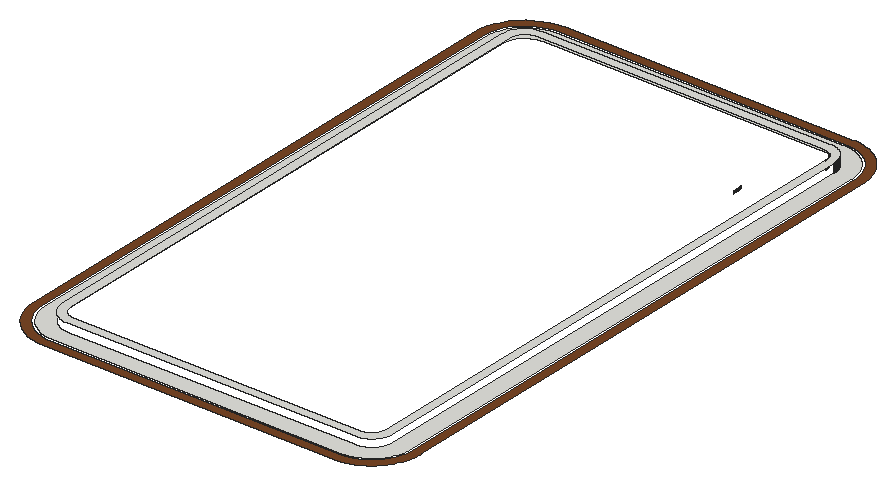
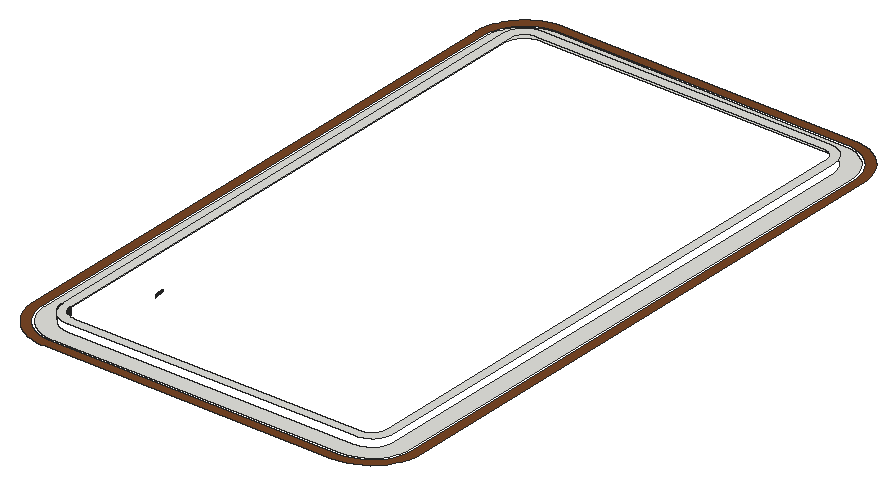
# SketchUp Ruby script. Lengths in inches.
U = 1.inch
M = Sketchup.active_model
def pt(a) = Geom::Point3d.new(a.map { |v| v * U })
def face(e, loops, mat)
  f = e.add_face(loops[0].map { |a| pt(a) })
  loops[1..].each { |l| e.add_face(l.map { |a| pt(a) }).erase! }
  f.material = f.back_material = mat if mat
  f
end
# faces: each face lists its corners as indices into pts; further lists are holes
def faces(e, pts, list, mat = nil) = list.each { |f| face(e, (f[0].is_a?(Array) ? f : [f]).map { |l| l.map { |i| pts[i] } }, mat) }
# xy, xz, yz: faces in a plane at the given z, y or x. An outline is a flat list of corners, or four numbers for a rectangle; further outlines are holes
def ring(l) = l.size == 4 ? [[l[0], l[1]], [l[2], l[1]], [l[2], l[3]], [l[0], l[3]]] : l.each_slice(2).to_a
def flat(e, list, mat, &to3) = list.each { |f| face(e, (f[0].is_a?(Array) ? f : [f]).map { |l| ring(l).map { |u, v| to3.(u, v) } }, mat) }
def xy(e, z, list, mat = nil) = flat(e, list, mat) { |x, y| [x, y, z] }
def xz(e, y, list, mat = nil) = flat(e, list, mat) { |x, z| [x, y, z] }
def yz(e, x, list, mat = nil) = flat(e, list, mat) { |y, z| [x, y, z] }
def lines(e, pts, list) = list.each { |a, b| e.add_line(pt(pts[a]), pt(pts[b])) }
# prism: a flat outline (further loops are holes) pulled along v
def prism(e, loops, v, mat = nil)
  f = face(e, loops, mat); d = Geom::Vector3d.new(v.map { |x| x * U })
  f.pushpull(f.normal.samedirection?(d) ? d.length : -d.length)
end
def box(e, o, s, mat = nil) = prism(e, [[o, [o[0] + s[0], o[1], o[2]], [o[0] + s[0], o[1] + s[1], o[2]], [o[0], o[1] + s[1], o[2]]]], [0, 0, s[2]], mat)
def at(x, y, z, deg = 0) = Geom::Transformation.translation(pt([x, y, z])) * Geom::Transformation.rotation(ORIGIN, Z_AXIS, deg.degrees)
def axes(o, x, y, z) = Geom::Transformation.new([*x, 0, *y, 0, *z, 0, *pt(o).to_a, 1])
def part(name) = M.definitions.add(name)
# library, detail: a bought-in or finely detailed component or shape, given as its bounding box
def library(name, o, s) = part(name).tap { |d| box(d.entities, o, s) }
def detail(e, o, s) = box(e.add_group.entities, o, s)
def put(e, d, t, mat = nil) = e.add_instance(d, t).tap { |i| i.material = mat if mat }
def group(e, t, mat = nil) = e.add_group.tap { |g| g.transformation = t; g.material = mat if mat }.entities
root = M.entities
M.materials.add("[Wood Veneer 01]3").color = [120, 70, 37]
xy(root,121,[[[75.09,29.75,144.24,29.75,144.36,29.76,144.48,29.76,144.6,29.77,144.73,29.78,144.97,29.8,145.09,29.8125,145.21,29.83,145.33,29.85,145.45,29.86,145.57,29.88,145.6875,29.9,145.8,29.93,145.92,29.95,146.16,30.01,146.28,30.03,146.39,30.07,146.63,30.13,146.74,30.17,146.86,30.2,146.97,30.24,147.09,30.28,147.31,30.36,147.43,30.41,147.54,30.45,148.09,30.7,148.2,30.76,148.31,30.8125,148.41,30.87,148.52,30.93,148.73,31.05,148.83,31.11,148.9375,31.18,149.04,31.24,149.14,31.31,149.24,31.375,149.34,31.45,149.4375,31.52,149.53,31.59,149.63,31.66,149.73,31.74,149.82,31.8125,149.91,31.89,150.01,31.97,150.1,32.05,150.1875,32.125,150.28,32.21,150.37,32.29,150.45,32.375,150.54,32.46,150.625,32.55,150.71,32.63,150.79,32.72,150.875,32.8125,150.95,32.9,151.03,32.99,151.11,33.09,151.1875,33.18,151.26,33.27,151.34,33.37,151.41,33.47,151.48,33.5625,151.55,33.66,151.625,33.76,151.69,33.86,151.76,33.96,151.82,34.0625,151.89,34.17,151.95,34.27,152.07,34.48,152.13,34.59,152.1875,34.69,152.24,34.8,152.3,34.91,152.55,35.46,152.59,35.57,152.64,35.69,152.72,35.91,152.76,36.03,152.8,36.14,152.83,36.26,152.87,36.37,152.93,36.61,152.97,36.72,152.99,36.84,153.05,37.08,153.07,37.2,153.1,37.3125,153.12,37.43,153.14,37.55,153.15,37.67,153.17,37.79,153.1875,37.91,153.2,38.03,153.22,38.27,153.23,38.4,153.24,38.52,153.24,38.64,153.25,38.76,153.25,171.24,153.24,171.36,153.24,171.48,153.23,171.6,153.22,171.73,153.2,171.97,153.1875,172.09,153.17,172.21,153.15,172.33,153.14,172.45,153.12,172.57,153.1,172.6875,153.07,172.8,153.05,172.92,152.99,173.16,152.97,173.28,152.93,173.39,152.87,173.63,152.83,173.74,152.8,173.86,152.76,173.97,152.72,174.09,152.64,174.31,152.59,174.43,152.55,174.54,152.3,175.09,152.24,175.2,152.1875,175.31,152.13,175.41,152.07,175.52,151.95,175.73,151.89,175.83,151.82,175.9375,151.76,176.04,151.69,176.14,151.625,176.24,151.55,176.34,151.48,176.4375,151.41,176.53,151.34,176.63,151.26,176.73,151.1875,176.82,151.11,176.91,151.03,177.01,150.95,177.1,150.875,177.1875,150.79,177.28,150.71,177.37,150.625,177.45,150.54,177.54,150.45,177.625,150.37,177.71,150.28,177.79,150.1875,177.875,150.1,177.95,150.01,178.03,149.91,178.11,149.82,178.1875,149.73,178.26,149.63,178.34,149.53,178.41,149.4375,178.48,149.34,178.55,149.24,178.625,149.14,178.69,149.04,178.76,148.9375,178.82,148.83,178.89,148.73,178.95,148.52,179.07,148.41,179.13,148.31,179.1875,148.2,179.24,148.09,179.3,147.54,179.55,147.43,179.59,147.31,179.64,147.09,179.72,146.97,179.76,146.86,179.8,146.74,179.83,146.63,179.87,146.39,179.93,146.28,179.97,146.16,179.99,145.92,180.05,145.8,180.07,145.6875,180.1,145.57,180.12,145.45,180.14,145.33,180.15,145.21,180.17,145.09,180.1875,144.97,180.2,144.73,180.22,144.6,180.23,144.48,180.24,144.36,180.24,144.24,180.25,75.09,180.25,73.79,180.17,72.61,179.93,71.46,179.54,70.38,179.01,69.37,178.33,68.46,177.54,67.67,176.63,66.99,175.62,66.46,174.54,66.07,173.39,65.83,172.21,65.75,170.91,65.75,39.09,65.83,37.79,66.07,36.61,66.46,35.46,66.99,34.38,67.67,33.37,68.46,32.46,69.37,31.67,70.38,30.99,71.46,30.46,72.61,30.07,73.79,29.83],[75.22,33.75,74.32,33.81,73.64,33.94,73,34.16,72.38,34.47,71.8125,34.85,71.3,35.3,70.85,35.8125,70.47,36.38,70.16,37,69.94,37.64,69.81,38.32,69.75,39.22,69.75,170.78,69.81,171.68,69.94,172.36,70.16,173,70.47,173.62,70.85,174.1875,71.3,174.7,71.8125,175.15,72.38,175.53,73,175.84,73.64,176.06,74.32,176.19,75.22,176.25,144.21,176.25,144.27,176.24,144.34,176.24,144.41,176.23,144.48,176.23,144.69,176.2,144.75,176.2,144.82,176.19,144.89,176.17,144.96,176.16,145.02,176.15,145.09,176.14,145.23,176.1,145.29,176.09,145.43,176.05,145.49,176.03,145.56,176.01,145.62,175.99,145.6875,175.97,145.75,175.95,145.82,175.93,145.88,175.9,145.95,175.875,146.01,175.85,146.07,175.82,146.14,175.8,146.44,175.65,146.51,175.61,146.57,175.58,146.625,175.55,146.68,175.51,146.74,175.48,146.86,175.4,146.92,175.37,146.97,175.33,147.09,175.25,147.14,175.21,147.2,175.16,147.3,175.08,147.36,175.04,147.41,174.99,147.46,174.95,147.51,174.9,147.5625,174.86,147.61,174.81,147.81,174.61,147.86,174.5625,147.9,174.51,147.95,174.46,147.99,174.41,148.04,174.36,148.08,174.3,148.16,174.2,148.21,174.14,148.25,174.09,148.33,173.97,148.37,173.92,148.4,173.86,148.48,173.74,148.51,173.68,148.55,173.625,148.58,173.57,148.61,173.51,148.65,173.44,148.8,173.14,148.82,173.07,148.85,173.01,148.875,172.95,148.9,172.88,148.93,172.82,148.95,172.75,148.97,172.6875,148.99,172.62,149.01,172.56,149.03,172.49,149.05,172.43,149.09,172.29,149.1,172.23,149.14,172.09,149.15,172.02,149.16,171.96,149.17,171.89,149.19,171.82,149.2,171.75,149.2,171.69,149.23,171.48,149.23,171.41,149.24,171.34,149.24,171.27,149.25,171.21,149.25,38.79,149.24,38.73,149.24,38.66,149.23,38.59,149.23,38.52,149.2,38.31,149.2,38.25,149.19,38.18,149.17,38.11,149.16,38.04,149.15,37.98,149.14,37.91,149.1,37.77,149.09,37.71,149.05,37.57,149.03,37.51,149.01,37.44,148.99,37.38,148.97,37.3125,148.95,37.25,148.93,37.18,148.9,37.12,148.875,37.05,148.85,36.99,148.82,36.93,148.8,36.86,148.65,36.56,148.61,36.49,148.58,36.43,148.55,36.375,148.51,36.32,148.48,36.26,148.4,36.14,148.37,36.08,148.33,36.03,148.25,35.91,148.21,35.86,148.16,35.8,148.08,35.7,148.04,35.64,147.99,35.59,147.95,35.54,147.9,35.49,147.86,35.4375,147.81,35.39,147.61,35.19,147.5625,35.14,147.51,35.1,147.46,35.05,147.41,35.01,147.36,34.96,147.3,34.92,147.2,34.84,147.14,34.79,147.09,34.75,146.97,34.67,146.92,34.63,146.86,34.6,146.74,34.52,146.68,34.49,146.625,34.45,146.57,34.42,146.51,34.39,146.44,34.35,146.14,34.2,146.07,34.18,146.01,34.15,145.95,34.125,145.88,34.1,145.82,34.07,145.75,34.05,145.6875,34.03,145.62,34.01,145.56,33.99,145.49,33.97,145.43,33.95,145.29,33.91,145.23,33.9,145.09,33.86,145.02,33.85,144.96,33.84,144.89,33.83,144.82,33.81,144.75,33.8,144.69,33.8,144.48,33.77,144.41,33.77,144.34,33.76,144.27,33.76,144.21,33.75]]])
xy(root,121,[[[75,27,144.3125,27,144.47,27.01,144.63,27.02,144.78,27.03,145.1,27.05,145.25,27.07,145.41,27.08,145.57,27.1,145.72,27.125,145.88,27.15,146.03,27.17,146.1875,27.2,146.34,27.23,146.49,27.26,146.65,27.3,146.8,27.33,146.95,27.37,147.11,27.41,147.41,27.49,147.86,27.64,148.01,27.6875,148.15,27.74,148.3,27.8,148.45,27.85,148.59,27.91,148.74,27.97,148.88,28.04,149.02,28.1,149.17,28.17,149.73,28.45,149.86,28.53,150,28.61,150.14,28.6875,150.27,28.77,150.4,28.85,150.54,28.9375,150.67,29.02,150.93,29.2,151.05,29.29,151.18,29.38,151.31,29.48,151.43,29.58,151.55,29.67,151.67,29.77,151.91,29.98,152.03,30.08,152.15,30.1875,152.26,30.3,152.375,30.4,152.49,30.51,152.6,30.625,152.7,30.74,152.8125,30.85,152.92,30.97,153.02,31.09,153.23,31.33,153.33,31.45,153.42,31.57,153.52,31.69,153.62,31.82,153.71,31.95,153.8,32.07,153.98,32.33,154.0625,32.46,154.15,32.6,154.23,32.73,154.3125,32.86,154.39,33,154.47,33.14,154.55,33.27,154.83,33.83,154.9,33.98,154.96,34.12,155.03,34.26,155.09,34.41,155.15,34.55,155.2,34.7,155.26,34.85,155.3125,34.99,155.36,35.14,155.51,35.59,155.59,35.89,155.63,36.05,155.67,36.2,155.7,36.35,155.74,36.51,155.77,36.66,155.8,36.8125,155.83,36.97,155.85,37.12,155.875,37.28,155.9,37.43,155.92,37.59,155.93,37.75,155.95,37.9,155.97,38.22,155.98,38.37,155.99,38.53,156,38.6875,156,171.3125,155.99,171.47,155.98,171.63,155.97,171.78,155.95,172.1,155.93,172.25,155.92,172.41,155.9,172.57,155.875,172.72,155.85,172.88,155.83,173.03,155.8,173.1875,155.77,173.34,155.74,173.49,155.7,173.65,155.67,173.8,155.63,173.95,155.59,174.11,155.51,174.41,155.36,174.86,155.3125,175.01,155.26,175.15,155.2,175.3,155.15,175.45,155.09,175.59,155.03,175.74,154.96,175.88,154.9,176.02,154.83,176.17,154.55,176.73,154.47,176.86,154.39,177,154.3125,177.14,154.23,177.27,154.15,177.4,154.0625,177.54,153.98,177.67,153.8,177.93,153.71,178.05,153.62,178.18,153.52,178.31,153.42,178.43,153.33,178.55,153.23,178.67,153.02,178.91,152.92,179.03,152.8125,179.15,152.7,179.26,152.6,179.375,152.49,179.49,152.375,179.6,152.26,179.7,152.15,179.8125,152.03,179.92,151.91,180.02,151.67,180.23,151.55,180.33,151.43,180.42,151.31,180.52,151.18,180.62,151.05,180.71,150.93,180.8,150.67,180.98,150.54,181.0625,150.4,181.15,150.27,181.23,150.14,181.3125,150,181.39,149.86,181.47,149.73,181.55,149.17,181.83,149.02,181.9,148.88,181.96,148.74,182.03,148.59,182.09,148.45,182.15,148.3,182.2,148.15,182.26,148.01,182.3125,147.86,182.36,147.41,182.51,147.11,182.59,146.95,182.63,146.8,182.67,146.65,182.7,146.49,182.74,146.34,182.77,146.1875,182.8,146.03,182.83,145.88,182.85,145.72,182.875,145.57,182.9,145.41,182.92,145.25,182.93,145.1,182.95,144.78,182.97,144.63,182.98,144.47,182.99,144.3125,183,75,183,73.43,182.9,71.89,182.59,70.41,182.09,69,181.39,67.69,180.52,66.51,179.49,65.48,178.31,64.61,177,63.91,175.59,63.41,174.11,63.1,172.57,63,171,63,39,63.1,37.43,63.41,35.89,63.91,34.41,64.61,33,65.48,31.69,66.51,30.51,67.69,29.48,69,28.61,70.41,27.91,71.89,27.41,73.43,27.1],[75.07,29,73.7,29.09,72.41,29.34,71.17,29.77,70,30.34,68.91,31.07,67.93,31.93,67.07,32.91,66.34,34,65.77,35.17,65.34,36.41,65.09,37.7,65,39.07,65,170.93,65.09,172.3,65.34,173.59,65.77,174.83,66.34,176,67.07,177.09,67.93,178.07,68.91,178.93,70,179.66,71.17,180.23,72.41,180.66,73.7,180.91,75.07,181,144.26,181,144.39,180.99,144.52,180.99,144.78,180.97,144.92,180.96,145.05,180.95,145.31,180.91,145.43,180.9,145.5625,180.875,145.69,180.86,145.82,180.83,145.95,180.81,146.21,180.75,146.33,180.72,146.59,180.66,146.71,180.625,146.84,180.59,146.97,180.55,147.21,180.47,147.34,180.43,147.46,180.38,147.58,180.34,147.71,180.29,147.83,180.24,147.95,180.1875,148.07,180.14,148.1875,180.08,148.31,180.03,148.42,179.97,148.66,179.85,148.77,179.79,148.89,179.72,149,179.66,149.11,179.59,149.22,179.53,149.34,179.46,149.45,179.39,149.56,179.31,149.66,179.24,149.77,179.17,149.88,179.09,149.98,179.01,150.09,178.93,150.29,178.77,150.39,178.6875,150.49,178.6,150.59,178.52,150.79,178.34,150.88,178.25,150.98,178.16,151.16,177.98,151.25,177.88,151.34,177.79,151.52,177.59,151.6,177.49,151.6875,177.39,151.77,177.29,151.93,177.09,152.01,176.98,152.09,176.88,152.17,176.77,152.24,176.66,152.31,176.56,152.39,176.45,152.46,176.34,152.53,176.22,152.59,176.11,152.66,176,152.72,175.89,152.79,175.77,152.85,175.66,152.97,175.42,153.03,175.31,153.08,175.1875,153.14,175.07,153.1875,174.95,153.24,174.83,153.29,174.71,153.34,174.58,153.38,174.46,153.43,174.34,153.47,174.21,153.55,173.97,153.59,173.84,153.625,173.71,153.66,173.59,153.72,173.33,153.75,173.21,153.81,172.95,153.83,172.82,153.86,172.69,153.875,172.5625,153.9,172.43,153.91,172.31,153.95,172.05,153.96,171.92,153.97,171.78,153.99,171.52,153.99,171.39,154,171.26,154,38.74,153.99,38.61,153.99,38.48,153.97,38.22,153.96,38.08,153.95,37.95,153.91,37.69,153.9,37.57,153.875,37.4375,153.86,37.31,153.83,37.18,153.81,37.05,153.75,36.79,153.72,36.67,153.66,36.41,153.625,36.29,153.59,36.16,153.55,36.03,153.47,35.79,153.43,35.66,153.38,35.54,153.34,35.42,153.29,35.29,153.24,35.17,153.1875,35.05,153.14,34.93,153.08,34.8125,153.03,34.69,152.97,34.58,152.85,34.34,152.79,34.23,152.72,34.11,152.66,34,152.59,33.89,152.53,33.78,152.46,33.66,152.39,33.55,152.31,33.44,152.24,33.34,152.17,33.23,152.09,33.12,152.01,33.02,151.93,32.91,151.77,32.71,151.6875,32.61,151.6,32.51,151.52,32.41,151.34,32.21,151.25,32.12,151.16,32.02,150.98,31.84,150.88,31.75,150.79,31.66,150.59,31.48,150.49,31.4,150.39,31.3125,150.29,31.23,150.09,31.07,149.98,30.99,149.88,30.91,149.77,30.83,149.66,30.76,149.56,30.69,149.45,30.61,149.34,30.54,149.22,30.47,149.11,30.41,149,30.34,148.89,30.28,148.77,30.21,148.66,30.15,148.42,30.03,148.31,29.97,148.1875,29.92,148.07,29.86,147.95,29.8125,147.83,29.76,147.71,29.71,147.58,29.66,147.46,29.62,147.34,29.57,147.21,29.53,146.97,29.45,146.84,29.41,146.71,29.375,146.59,29.34,146.33,29.28,146.21,29.25,145.95,29.19,145.82,29.17,145.69,29.14,145.5625,29.125,145.43,29.1,145.31,29.09,145.05,29.05,144.92,29.04,144.78,29.03,144.52,29.01,144.39,29.01,144.26,29]]],"[Wood Veneer 01]3")
xy(root,123,[[[75.22,33.75,144.21,33.75,144.27,33.76,144.34,33.76,144.41,33.77,144.48,33.77,144.69,33.8,144.75,33.8,144.82,33.81,144.89,33.83,144.96,33.84,145.02,33.85,145.09,33.86,145.23,33.9,145.29,33.91,145.43,33.95,145.49,33.97,145.56,33.99,145.62,34.01,145.6875,34.03,145.75,34.05,145.82,34.07,145.88,34.1,145.95,34.125,146.01,34.15,146.07,34.18,146.14,34.2,146.44,34.35,146.51,34.39,146.57,34.42,146.625,34.45,146.68,34.49,146.74,34.52,146.86,34.6,146.92,34.63,146.97,34.67,147.09,34.75,147.14,34.79,147.2,34.84,147.3,34.92,147.36,34.96,147.41,35.01,147.46,35.05,147.51,35.1,147.5625,35.14,147.61,35.19,147.81,35.39,147.86,35.4375,147.9,35.49,147.95,35.54,147.99,35.59,148.04,35.64,148.08,35.7,148.16,35.8,148.21,35.86,148.25,35.91,148.33,36.03,148.37,36.08,148.4,36.14,148.48,36.26,148.51,36.32,148.55,36.375,148.58,36.43,148.61,36.49,148.65,36.56,148.8,36.86,148.82,36.93,148.85,36.99,148.875,37.05,148.9,37.12,148.93,37.18,148.95,37.25,148.97,37.3125,148.99,37.38,149.01,37.44,149.03,37.51,149.05,37.57,149.09,37.71,149.1,37.77,149.14,37.91,149.15,37.98,149.16,38.04,149.17,38.11,149.19,38.18,149.2,38.25,149.2,38.31,149.23,38.52,149.23,38.59,149.24,38.66,149.24,38.73,149.25,38.79,149.25,171.21,149.24,171.27,149.24,171.34,149.23,171.41,149.23,171.48,149.2,171.69,149.2,171.75,149.19,171.82,149.17,171.89,149.16,171.96,149.15,172.02,149.14,172.09,149.1,172.23,149.09,172.29,149.05,172.43,149.03,172.49,149.01,172.56,148.99,172.62,148.97,172.6875,148.95,172.75,148.93,172.82,148.9,172.88,148.875,172.95,148.85,173.01,148.82,173.07,148.8,173.14,148.65,173.44,148.61,173.51,148.58,173.57,148.55,173.625,148.51,173.68,148.48,173.74,148.4,173.86,148.37,173.92,148.33,173.97,148.25,174.09,148.21,174.14,148.16,174.2,148.08,174.3,148.04,174.36,147.99,174.41,147.95,174.46,147.9,174.51,147.86,174.5625,147.81,174.61,147.61,174.81,147.5625,174.86,147.51,174.9,147.46,174.95,147.41,174.99,147.36,175.04,147.3,175.08,147.2,175.16,147.14,175.21,147.09,175.25,146.97,175.33,146.92,175.37,146.86,175.4,146.74,175.48,146.68,175.51,146.625,175.55,146.57,175.58,146.51,175.61,146.44,175.65,146.14,175.8,146.07,175.82,146.01,175.85,145.95,175.875,145.88,175.9,145.82,175.93,145.75,175.95,145.6875,175.97,145.62,175.99,145.56,176.01,145.49,176.03,145.43,176.05,145.29,176.09,145.23,176.1,145.09,176.14,145.02,176.15,144.96,176.16,144.89,176.17,144.82,176.19,144.75,176.2,144.69,176.2,144.48,176.23,144.41,176.23,144.34,176.24,144.27,176.24,144.21,176.25,75.22,176.25,74.32,176.19,73.64,176.06,73,175.84,72.38,175.53,71.8125,175.15,71.3,174.7,70.85,174.1875,70.47,173.62,70.16,173,69.94,172.36,69.81,171.68,69.75,170.78,69.75,39.22,69.81,38.32,69.94,37.64,70.16,37,70.47,36.38,70.85,35.8125,71.3,35.3,71.8125,34.85,72.38,34.47,73,34.16,73.64,33.94,74.32,33.81],[75.29,35.75,74.58,35.8,74.16,35.88,73.76,36.01,73.38,36.2,73.03,36.4375,72.72,36.72,72.4375,37.03,72.2,37.38,72.01,37.76,71.88,38.16,71.8,38.58,71.75,39.29,71.75,170.71,71.8,171.42,71.88,171.84,72.01,172.24,72.2,172.62,72.4375,172.97,72.72,173.28,73.03,173.5625,73.38,173.8,73.76,173.99,74.16,174.12,74.58,174.2,75.29,174.25,144.17,174.25,144.21,174.24,144.3,174.24,144.34,174.23,144.38,174.23,144.42,174.22,144.47,174.22,144.55,174.2,144.59,174.2,144.63,174.1875,144.68,174.18,144.92,174.12,144.96,174.1,145.04,174.08,145.08,174.0625,145.125,174.05,145.16,174.03,145.2,174.02,145.24,174,145.28,173.99,145.4,173.93,145.4375,173.91,145.48,173.9,145.51,173.875,145.55,173.86,145.59,173.84,145.625,173.8125,145.66,173.79,145.7,173.77,145.73,173.75,145.77,173.73,145.81,173.7,145.84,173.68,145.875,173.65,145.91,173.63,145.94,173.6,145.98,173.58,146.01,173.55,146.05,173.53,146.14,173.44,146.17,173.42,146.21,173.39,146.39,173.21,146.42,173.17,146.44,173.14,146.53,173.05,146.55,173.01,146.58,172.98,146.6,172.94,146.63,172.91,146.65,172.875,146.68,172.84,146.7,172.81,146.73,172.77,146.75,172.73,146.77,172.7,146.79,172.66,146.8125,172.625,146.84,172.59,146.86,172.55,146.875,172.51,146.9,172.48,146.91,172.4375,146.93,172.4,146.99,172.28,147,172.24,147.02,172.2,147.03,172.16,147.05,172.125,147.0625,172.08,147.08,172.04,147.1,171.96,147.12,171.92,147.18,171.68,147.1875,171.63,147.2,171.59,147.2,171.55,147.22,171.47,147.22,171.42,147.23,171.38,147.23,171.34,147.24,171.3,147.24,171.21,147.25,171.17,147.25,38.83,147.24,38.79,147.24,38.7,147.23,38.66,147.23,38.62,147.22,38.58,147.22,38.53,147.2,38.45,147.2,38.41,147.1875,38.37,147.18,38.32,147.12,38.08,147.1,38.04,147.08,37.96,147.0625,37.92,147.05,37.875,147.03,37.84,147.02,37.8,147,37.76,146.99,37.72,146.93,37.6,146.91,37.5625,146.9,37.52,146.875,37.49,146.86,37.45,146.84,37.41,146.8125,37.375,146.79,37.34,146.77,37.3,146.75,37.27,146.73,37.23,146.7,37.19,146.68,37.16,146.65,37.125,146.63,37.09,146.6,37.06,146.58,37.02,146.55,36.99,146.53,36.95,146.44,36.86,146.42,36.83,146.39,36.79,146.21,36.61,146.17,36.58,146.14,36.56,146.05,36.47,146.01,36.45,145.98,36.42,145.94,36.4,145.91,36.37,145.875,36.35,145.84,36.32,145.81,36.3,145.77,36.27,145.73,36.25,145.7,36.23,145.66,36.21,145.625,36.1875,145.59,36.16,145.55,36.14,145.51,36.125,145.48,36.1,145.4375,36.09,145.4,36.07,145.28,36.01,145.24,36,145.2,35.98,145.16,35.97,145.125,35.95,145.08,35.9375,145.04,35.92,144.96,35.9,144.92,35.88,144.68,35.82,144.63,35.8125,144.59,35.8,144.55,35.8,144.47,35.78,144.42,35.78,144.38,35.77,144.34,35.77,144.3,35.76,144.21,35.76,144.17,35.75]]])
yz(root,139.5,[[153,121,153.18,121.5],[153.18,121,153.35,121.5]],"[Wood Veneer 01]3")
yz(root,147.2,[[171.55,121,171.59,123]])
yz(root,147.22,[[171.42,121,171.47,123]])
yz(root,147.23,[[171.34,121,171.38,123]])
yz(root,147.24,[[171.21,121,171.25,123],[171.25,121,171.3,123]])
yz(root,147.25,[[170.97,121,171.04,123],[171.04,121,171.09,123],[171.09,121,171.13,123],[171.13,121,171.17,123]])
yz(root,149.2,[[171.69,121,171.75,123]])
yz(root,149.23,[[171.41,121,171.48,123]])
yz(root,149.24,[[171.27,121,171.34,123]])
yz(root,149.25,[[170.98,121,171.07,123],[171.07,121,171.14,123],[171.14,121,171.21,123]])
p = [[139.5,153.35,121],[139.49,153.53,121],[139.49,153.53,121.5],[139.5,153.35,121.5],[139.48,153.71,121],[139.48,153.71,121.5],
  [139.47,153.88,121],[139.47,153.88,121.5],[139.46,154.06,121],[139.46,154.06,121.5],[139.44,154.24,121],[139.44,154.24,121.5],
  [139.43,154.41,121],[139.43,154.41,121.5],[139.41,154.59,121],[139.41,154.59,121.5],[139.38,154.76,121],[139.38,154.76,121.5],
  [139.36,154.9375,121],[139.36,154.9375,121.5],[139.33,155.11,121],[139.33,155.11,121.5],[139.31,155.29,121],[139.31,155.29,121.5],
  [139.27,155.46,121],[139.27,155.46,121.5],[139.24,155.63,121],[139.24,155.63,121.5],[147.24,171.21,121],[147.25,171.17,121],
  [147.25,171.17,123],[147.24,171.21,123],[149.25,171.21,121],[149.24,171.27,121],[149.24,171.27,123],[149.25,171.21,123],
  [147.23,171.34,121],[147.24,171.3,121],[147.24,171.3,123],[147.23,171.34,123],[149.24,171.34,121],[149.23,171.41,121],
  [149.23,171.41,123],[149.24,171.34,123],[147.22,171.42,121],[147.23,171.38,121],[147.23,171.38,123],[147.22,171.42,123],
  [147.21,171.51,121],[147.22,171.47,121],[147.22,171.47,123],[147.21,171.51,123],[147.2,171.55,121],[147.2,171.55,123],
  [149.23,171.48,121],[149.22,171.55,121],[149.22,171.55,123],[149.23,171.48,123],[149.21,171.62,121],[149.21,171.62,123],
  [147.1875,171.63,121],[147.2,171.59,121],[147.2,171.59,123],[147.1875,171.63,123],[147.18,171.68,121],[147.18,171.68,123],
  [149.2,171.69,121],[149.2,171.69,123],[147.17,171.72,121],[147.17,171.72,123],[147.16,171.76,121],[147.16,171.76,123],
  [147.15,171.8,121],[147.15,171.8,123],[147.14,171.84,121],[147.14,171.84,123],[147.13,171.88,121],[147.13,171.88,123],
  [149.2,171.75,121],[149.19,171.82,121],[149.19,171.82,123],[149.2,171.75,123],[149.17,171.89,121],[149.17,171.89,123],
  [147.12,171.92,121],[147.12,171.92,123],[147.1,171.96,121],[147.1,171.96,123],[149.16,171.96,121],[149.16,171.96,123],
  [147.09,172,121],[147.09,172,123],[147.08,172.04,121],[147.08,172.04,123],[147.0625,172.08,121],[147.0625,172.08,123],
  [149.15,172.02,121],[149.15,172.02,123],[149.14,172.09,121],[149.14,172.09,123],[147.05,172.125,121],[147.05,172.125,123],
  [147.03,172.16,121],[147.03,172.16,123],[149.12,172.16,121],[149.12,172.16,123],[147.02,172.2,121],[147.02,172.2,123],
  [147,172.24,121],[147,172.24,123],[146.99,172.28,121],[146.99,172.28,123],[149.1,172.23,121],[149.1,172.23,123],
  [149.09,172.29,121],[149.09,172.29,123],[146.97,172.32,121],[146.97,172.32,123],[146.95,172.36,121],[146.95,172.36,123],
  [149.07,172.36,121],[149.07,172.36,123],[146.93,172.4,121],[146.93,172.4,123],[146.91,172.4375,121],[146.91,172.4375,123],
  [146.9,172.48,121],[146.9,172.48,123],[149.05,172.43,121],[149.03,172.49,121],[149.03,172.49,123],[149.05,172.43,123],
  [146.875,172.51,121],[146.875,172.51,123],[146.86,172.55,121],[146.86,172.55,123],[149.01,172.56,121],[149.01,172.56,123],
  [146.84,172.59,121],[146.84,172.59,123],[146.8125,172.625,121],[146.8125,172.625,123],[146.79,172.66,121],[146.79,172.66,123],
  [148.99,172.62,121],[148.99,172.62,123],[148.97,172.6875,121],[148.97,172.6875,123],[146.75,172.73,121],[146.77,172.7,121],
  [146.77,172.7,123],[146.75,172.73,123],[146.73,172.77,121],[146.73,172.77,123],[148.95,172.75,121],[148.95,172.75,123],
  [146.7,172.81,121],[146.7,172.81,123],[146.68,172.84,121],[146.68,172.84,123],[146.65,172.875,121],[146.65,172.875,123],
  [148.93,172.82,121],[148.93,172.82,123],[148.9,172.88,121],[148.9,172.88,123],[146.63,172.91,121],[146.63,172.91,123],
  [146.6,172.94,121],[146.6,172.94,123],[146.58,172.98,121],[146.58,172.98,123],[148.875,172.95,121],[148.875,172.95,123],
  [148.85,173.01,121],[148.85,173.01,123],[146.53,173.05,121],[146.55,173.01,121],[146.55,173.01,123],[146.53,173.05,123],
  [146.5,173.08,121],[146.5,173.08,123],[148.82,173.07,121],[148.82,173.07,123],[146.44,173.14,121],[146.47,173.11,121],
  [146.47,173.11,123],[146.44,173.14,123],[146.42,173.17,121],[146.42,173.17,123],[148.8,173.14,121],[148.8,173.14,123],
  [148.77,173.2,121],[148.77,173.2,123],[146.33,173.27,121],[146.36,173.24,121],[146.36,173.24,123],[146.33,173.27,123],
  [146.39,173.21,121],[146.39,173.21,123],[148.74,173.26,121],[148.74,173.26,123],[146.24,173.36,121],[146.27,173.33,121],
  [146.27,173.33,123],[146.24,173.36,123],[146.3,173.3,121],[146.3,173.3,123],[148.71,173.32,121],[148.71,173.32,123],
  [148.68,173.38,121],[148.68,173.38,123],[146.14,173.44,121],[146.17,173.42,121],[146.17,173.42,123],[146.14,173.44,123],
  [146.11,173.47,121],[146.11,173.47,123],[146.21,173.39,121],[146.21,173.39,123],[148.65,173.44,121],[148.65,173.44,123],
  [148.61,173.51,121],[148.61,173.51,123],[146.05,173.53,121],[146.08,173.5,121],[146.08,173.5,123],[146.05,173.53,123],
  [146.01,173.55,121],[146.01,173.55,123],[148.58,173.57,121],[148.58,173.57,123],[145.94,173.6,121],[145.98,173.58,121],
  [145.98,173.58,123],[145.94,173.6,123],[148.55,173.625,121],[148.55,173.625,123]]
faces(root,p,[[0,1,2,3],[1,4,5,2],[4,6,7,5],[6,8,9,7],[8,10,11,9],[10,12,13,11],[12,14,15,13],[14,16,17,15],
  [16,18,19,17],[18,20,21,19],[20,22,23,21],[22,24,25,23],[24,26,27,25]],"[Wood Veneer 01]3")
faces(root,p,[[28,29,30,31],[32,33,34,35],[36,37,38,39],[40,41,42,43],[44,45,46,47],[48,49,50,51],[52,48,51,53],[54,55,56,57],
  [55,58,59,56],[60,61,62,63],[64,60,63,65],[58,66,67,59],[68,64,65,69],[70,68,69,71],[72,70,71,73],[74,72,73,75],
  [76,74,75,77],[78,79,80,81],[79,82,83,80],[84,76,77,85],[86,84,85,87],[82,88,89,83],[90,86,87,91],[92,90,91,93],
  [94,92,93,95],[88,96,97,89],[96,98,99,97],[100,94,95,101],[102,100,101,103],[98,104,105,99],[106,102,103,107],[108,106,107,109],
  [110,108,109,111],[104,112,113,105],[112,114,115,113],[116,110,111,117],[118,116,117,119],[114,120,121,115],[122,118,119,123],[124,122,123,125],
  [126,124,125,127],[128,129,130,131],[120,128,131,121],[132,126,127,133],[134,132,133,135],[129,136,137,130],[138,134,135,139],[140,138,139,141],
  [142,140,141,143],[136,144,145,137],[144,146,147,145],[148,149,150,151],[152,148,151,153],[149,142,143,150],[146,154,155,147],[156,152,153,157],
  [158,156,157,159],[160,158,159,161],[154,162,163,155],[162,164,165,163],[166,160,161,167],[168,166,167,169],[170,168,169,171],[164,172,173,165],
  [172,174,175,173],[176,177,178,179],[180,176,179,181],[177,170,171,178],[174,182,183,175],[184,185,186,187],[188,184,187,189],[185,180,181,186],
  [182,190,191,183],[190,192,193,191],[194,195,196,197],[198,188,189,199],[195,198,199,196],[192,200,201,193],[202,203,204,205],[206,194,197,207],
  [203,206,207,204],[200,208,209,201],[208,210,211,209],[212,213,214,215],[216,212,215,217],[218,202,205,219],[213,218,219,214],[210,220,221,211],
  [220,222,223,221],[224,225,226,227],[228,224,227,229],[225,216,217,226],[222,230,231,223],[232,233,234,235],[233,228,229,234],[230,236,237,231]])
